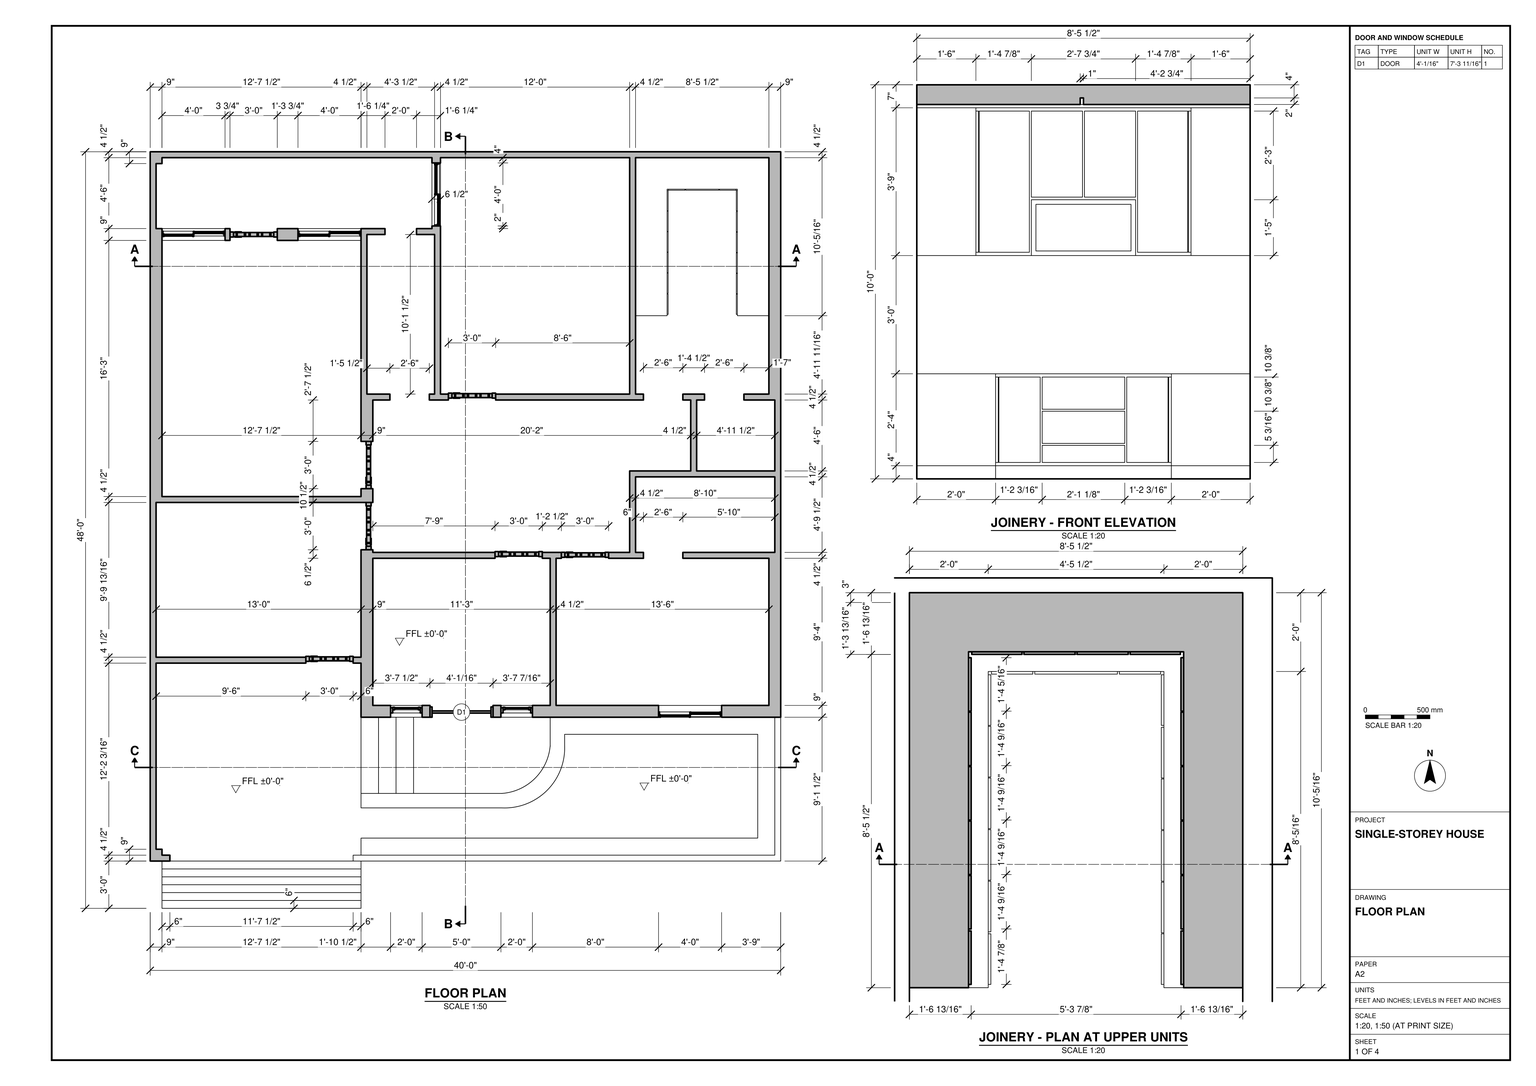
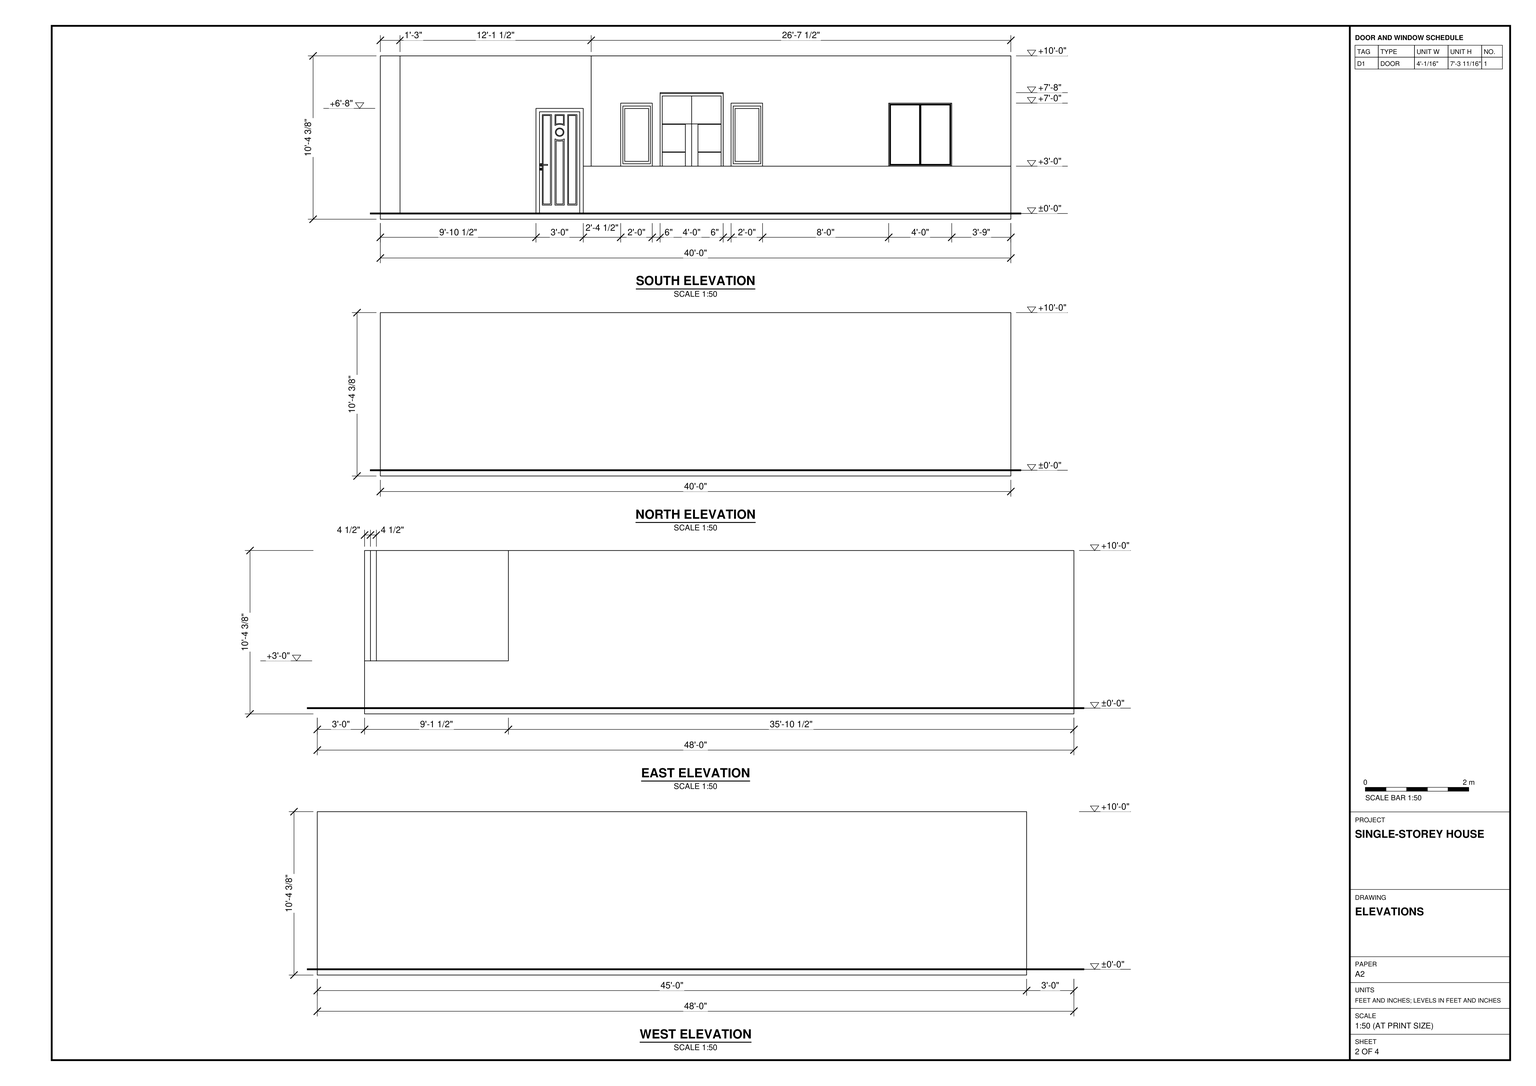
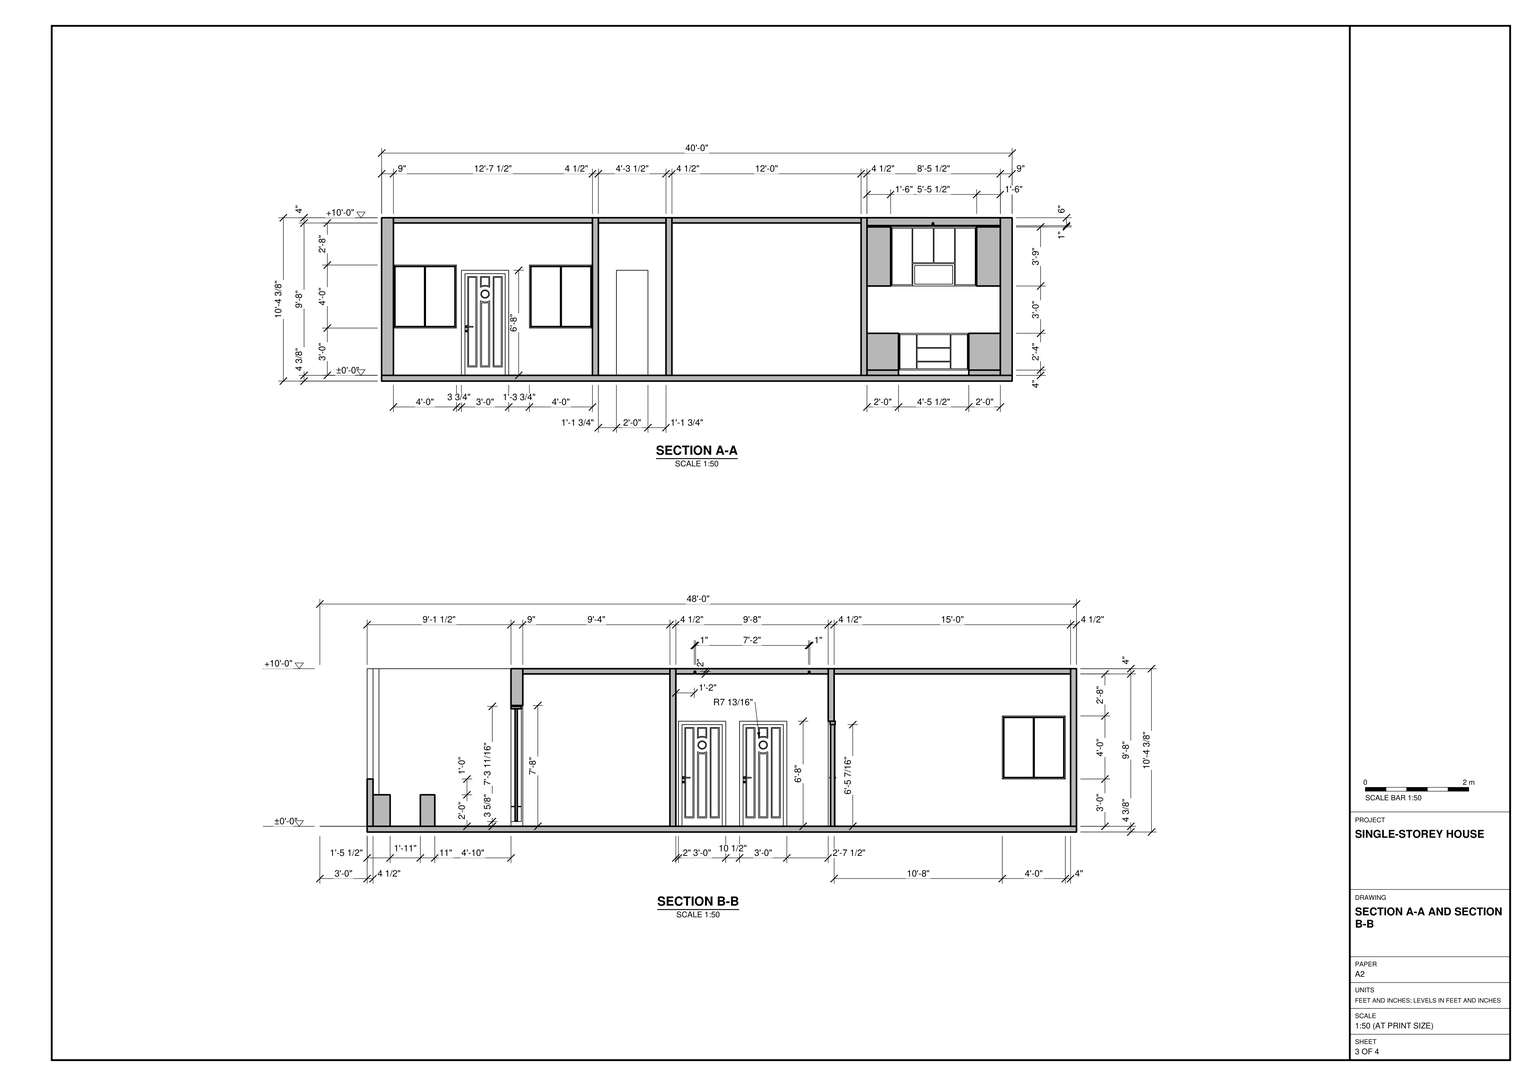
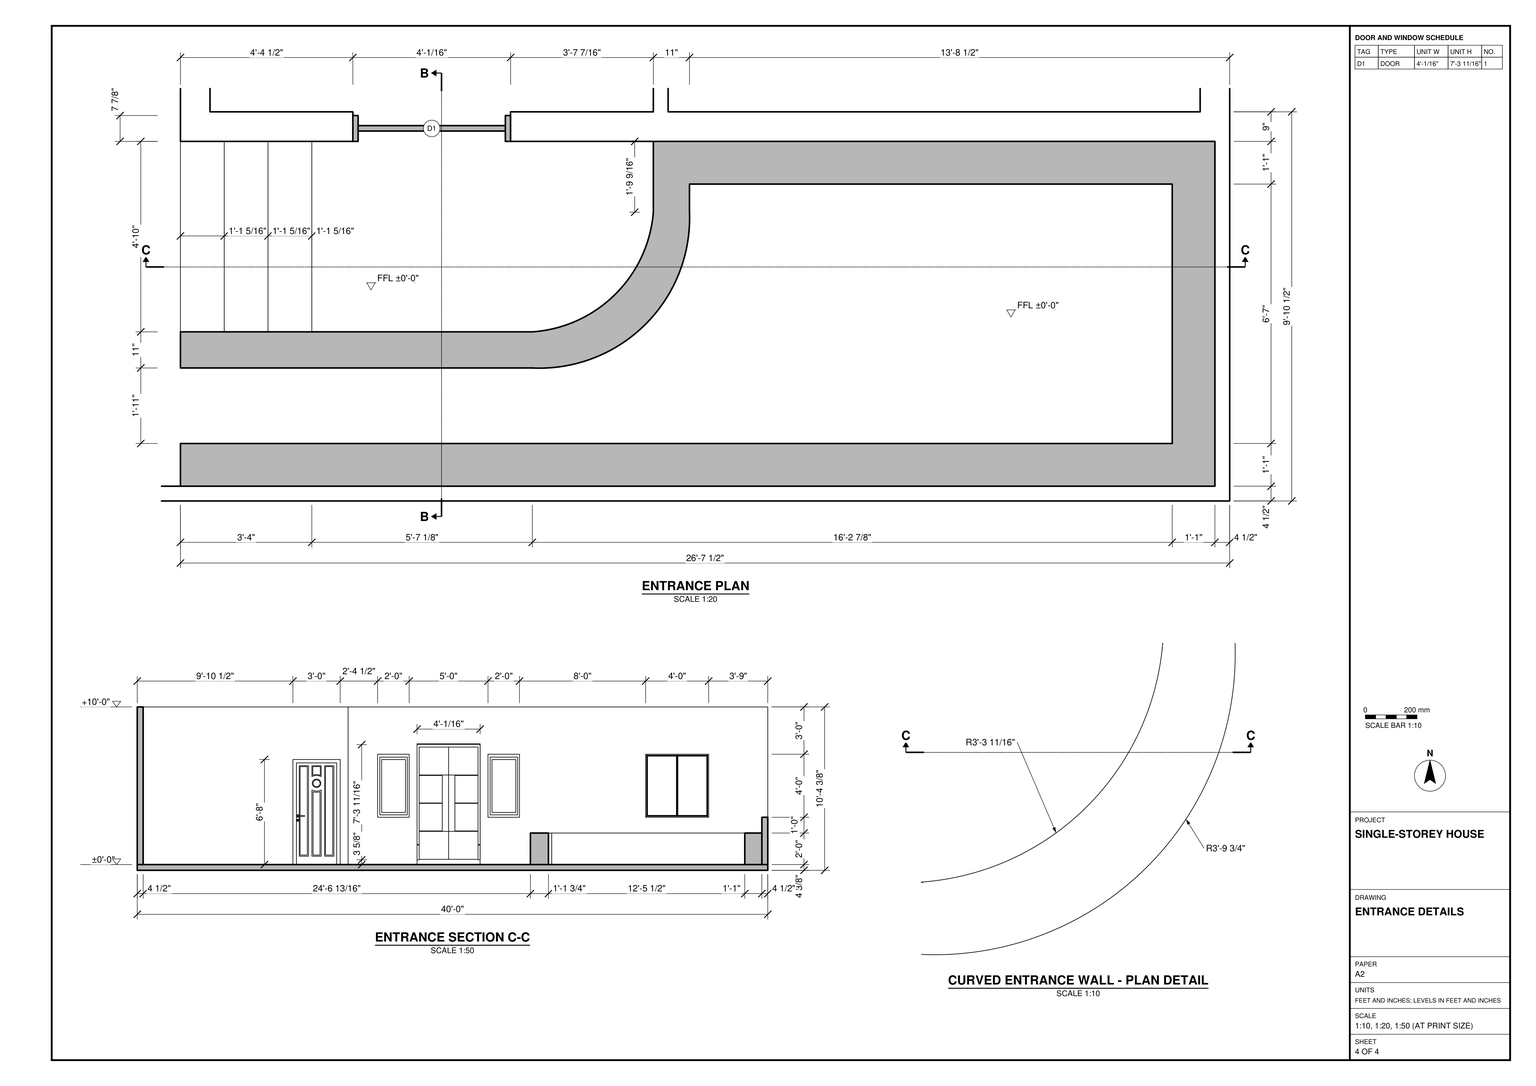
Build the house in SketchUp from task_files/diagram_01.pdf. Work in feet and inches. The overall dimensions, including the entry steps, are 40'-0" east to west, 48'-0" north to south and 10'-4 3/8" from the underside of the floor slab to the top of the roof. Use ±0'-0" as the finished floor level for the single storey.

Lay out the exterior walls and interior partitions from the floor plan, following the marked wall thicknesses rather than using one thickness throughout. Preserve the central circulation space, the rooms opening off it and the smaller compartments along the east side. Model the floor slab and flat roof slab using the sections. At the south entrance, include the steps on the west side and the low enclosure with its curved return. Fit the doors and framed window units to their openings, using the plan for placement and the elevations and sections for sill and head heights.

Build the joinery in the northeast room. Use the upper-unit plan for its U-shaped footprint and the front elevation for the upper cupboards, clear space above the base units and central drawer stack. Keep walls, slabs, roof and each furniture or joinery piece in separate groups or components, and use components for repeated parts. Decor and loose items shown may be represented by any suitable library components. Save one SketchUp model as output_files/single_storey_house_with_u_shaped_joinery.skp.

# SketchUp Ruby script. Lengths in inches.
U = 1.inch
M = Sketchup.active_model
def pt(a) = Geom::Point3d.new(a.map { |v| v * U })
def face(e, loops, mat)
  f = e.add_face(loops[0].map { |a| pt(a) })
  loops[1..].each { |l| e.add_face(l.map { |a| pt(a) }).erase! }
  f.material = f.back_material = mat if mat
  f
end
# faces: each face lists its corners as indices into pts; further lists are holes
def faces(e, pts, list, mat = nil) = list.each { |f| face(e, (f[0].is_a?(Array) ? f : [f]).map { |l| l.map { |i| pts[i] } }, mat) }
# xy, xz, yz: faces in a plane at the given z, y or x. An outline is a flat list of corners, or four numbers for a rectangle; further outlines are holes
def ring(l) = l.size == 4 ? [[l[0], l[1]], [l[2], l[1]], [l[2], l[3]], [l[0], l[3]]] : l.each_slice(2).to_a
def flat(e, list, mat, &to3) = list.each { |f| face(e, (f[0].is_a?(Array) ? f : [f]).map { |l| ring(l).map { |u, v| to3.(u, v) } }, mat) }
def xy(e, z, list, mat = nil) = flat(e, list, mat) { |x, y| [x, y, z] }
def xz(e, y, list, mat = nil) = flat(e, list, mat) { |x, z| [x, y, z] }
def yz(e, x, list, mat = nil) = flat(e, list, mat) { |y, z| [x, y, z] }
def lines(e, pts, list) = list.each { |a, b| e.add_line(pt(pts[a]), pt(pts[b])) }
# prism: a flat outline (further loops are holes) pulled along v
def prism(e, loops, v, mat = nil)
  f = face(e, loops, mat); d = Geom::Vector3d.new(v.map { |x| x * U })
  f.pushpull(f.normal.samedirection?(d) ? d.length : -d.length)
end
def box(e, o, s, mat = nil) = prism(e, [[o, [o[0] + s[0], o[1], o[2]], [o[0] + s[0], o[1] + s[1], o[2]], [o[0], o[1] + s[1], o[2]]]], [0, 0, s[2]], mat)
def at(x, y, z, deg = 0) = Geom::Transformation.translation(pt([x, y, z])) * Geom::Transformation.rotation(ORIGIN, Z_AXIS, deg.degrees)
def axes(o, x, y, z) = Geom::Transformation.new([*x, 0, *y, 0, *z, 0, *pt(o).to_a, 1])
def part(name) = M.definitions.add(name)
# library, detail: a bought-in or finely detailed component or shape, given as its bounding box
def library(name, o, s) = part(name).tap { |d| box(d.entities, o, s) }
def detail(e, o, s) = box(e.add_group.entities, o, s)
def put(e, d, t, mat = nil) = e.add_instance(d, t).tap { |i| i.material = mat if mat }
def group(e, t, mat = nil) = e.add_group.tap { |g| g.transformation = t; g.material = mat if mat }.entities
root = M.entities
M.materials.add("[0128_White]1").color = [255, 255, 255]
c1 = library("Double Door-006",[0,-7.875,0],[59.06,7.875,92.52])
c2 = library("door58",[0,0,0],[34.0625,4.69,80])
c3 = library("PENTEK_RP+Fineline+50S_Sliding_Door+(1)",[0,-2.27,-0.09],[99.27,4.05,99.27])
c4 = library("Group\#35",[29.18,0,0],[33.81,4.33,51.18])
c5 = library("Group\#7",[-0.5,-0.5,-0.1],[168.5,89,0.2])
c6 = library("Group\#8",[-0.5,-0.5,-0.1],[33.5,27,0.2])
c7 = library("Group\#5",[0,0,0],[101.5,120.3,28])
c8 = library("Group\#3",[0,0,0],[101.5,120.3,45])
c9 = library("Group\#11",[-0.5,-0.5,-6],[102.5,181,6])
xy(root,0,[[9,0,160.5,6],[9,6,160.5,12],[9,12,160.5,18],[9,18,160.5,24],[9,24,160.5,30],
  [9,30,160.5,36],[160.5,40.5,475.5,40.5,475.5,145.5,304.5,145.5,304.5,123.9375,315.5,123.9375,315.5,132.5,462.5,132.5,462.5,53.5,160.5,53.5],[273.77,86.84,273.15,86.85,272.53,86.87,271.92,86.91,271.3,86.95,270.68,87.01,270.07,87.09,269.45,87.17,268.84,87.27,268.23,87.38,267.625,87.5,268.19,87.54,268.76,87.59,269.33,87.65,269.9,87.72,270.46,87.8,271.03,87.88,271.59,87.97,272.15,88.07,272.71,88.18,273.83,88.42,274.38,88.55,274.93,88.69,275.49,88.84,276.03,89,276.58,89.16,277.125,89.33,277.67,89.51,278.21,89.7,278.74,89.89,279.28,90.1,279.81,90.31,280.33,90.52,280.86,90.75,281.38,90.98,281.9,91.22,282.92,91.72,283.43,91.99,284.43,92.53,285.41,93.11,285.9,93.41,286.38,93.71,286.86,94.02,287.33,94.34,288.27,95,288.72,95.34,289.18,95.68,289.63,96.03,290.07,96.39,290.51,96.76,290.94,97.13,291.8,97.89,292.21,98.28,292.625,98.67,293.03,99.07,293.43,99.48,293.82,99.89,294.21,100.3125,294.59,100.73,294.97,101.16,295.34,101.6,295.7,102.04,296.0625,102.48,296.41,102.93,296.76,103.39,297.09,103.85,297.42,104.3125,297.75,104.78,298.07,105.26,298.375,105.73,298.68,106.22,298.98,106.7,299.27,107.2,299.55,107.69,299.83,108.19,300.09,108.69,300.61,109.71,300.86,110.23,301.09,110.75,301.33,111.27,301.55,111.79,301.77,112.32,301.97,112.85,302.18,113.38,302.56,114.46,302.73,115,302.9,115.55,303.07,116.09,303.37,117.19,303.51,117.75,303.64,118.3,303.76,118.86,303.875,119.42,303.98,119.98,304.08,120.54,304.17,121.1,304.25,121.67,304.33,122.23,304.45,123.37,304.5,123.9375,304.61,123.33,304.72,122.72,304.81,122.11,304.88,121.49,304.95,120.875,305,120.26,305.04,119.64,305.07,119.02,305.09,118.4,305.09,117.78,305.08,117.16,305.0625,116.54,305.03,115.93,304.98,115.31,304.92,114.69,304.85,114.08,304.77,113.46,304.68,112.85,304.57,112.24,304.45,111.63,304.32,111.03,304.18,110.42,304.02,109.82,303.68,108.64,303.28,107.46,303.07,106.88,302.84,106.3,302.61,105.73,302.36,105.16,302.1,104.6,301.83,104.04,301.55,103.49,300.95,102.41,300.63,101.87,300.31,101.35,299.97,100.82,299.63,100.3125,299.27,99.8,298.91,99.3,298.53,98.8125,298.15,98.33,297.75,97.85,297.35,97.38,296.93,96.92,296.51,96.47,296.08,96.02,295.64,95.59,295.1875,95.16,294.73,94.74,294.26,94.34,293.79,93.9375,293.31,93.55,292.82,93.17,292.32,92.8,291.82,92.4375,291.31,92.09,290.79,91.75,290.27,91.42,289.73,91.1,289.2,90.79,288.1,90.21,287.55,89.94,286.99,89.67,286.42,89.42,285.85,89.18,285.28,88.95,284.7,88.73,284.12,88.52,283.53,88.33,282.9375,88.14,282.34,87.97,281.74,87.81,281.14,87.66,280.54,87.53,279.93,87.4,279.32,87.29,278.71,87.19,278.1,87.1,277.48,87.03,276.87,86.97,276.25,86.91,275.63,86.875,275.01,86.85,274.39,86.84],[160.5,87.5,173.83,145.5],[173.83,87.5,187.17,145.5],
  [187.17,87.5,200.5,145.5]])
xy(root,24,[[160.5,40.5,475.5,40.5,475.5,145.5,304.5,145.5,304.5,123.9375,304.45,123.37,304.33,122.23,304.25,121.67,304.17,121.1,304.08,120.54,303.98,119.98,303.875,119.42,303.76,118.86,303.64,118.3,303.51,117.75,303.37,117.19,303.07,116.09,302.9,115.55,302.73,115,302.56,114.46,302.18,113.38,301.97,112.85,301.77,112.32,301.55,111.79,301.33,111.27,301.09,110.75,300.86,110.23,300.61,109.71,300.09,108.69,299.83,108.19,299.55,107.69,299.27,107.2,298.98,106.7,298.68,106.22,298.375,105.73,298.07,105.26,297.75,104.78,297.42,104.3125,297.09,103.85,296.76,103.39,296.41,102.93,296.0625,102.48,295.7,102.04,295.34,101.6,294.97,101.16,294.59,100.73,294.21,100.3125,293.82,99.89,293.43,99.48,293.03,99.07,292.625,98.67,292.21,98.28,291.8,97.89,290.94,97.13,290.51,96.76,290.07,96.39,289.63,96.03,289.18,95.68,288.72,95.34,288.27,95,287.33,94.34,286.86,94.02,286.38,93.71,285.9,93.41,285.41,93.11,284.43,92.53,283.43,91.99,282.92,91.72,281.9,91.22,281.38,90.98,280.86,90.75,280.33,90.52,279.81,90.31,279.28,90.1,278.74,89.89,278.21,89.7,277.67,89.51,277.125,89.33,276.58,89.16,276.03,89,275.49,88.84,274.93,88.69,274.38,88.55,273.83,88.42,272.71,88.18,272.15,88.07,271.59,87.97,271.03,87.88,270.46,87.8,269.9,87.72,269.33,87.65,268.76,87.59,268.19,87.54,267.625,87.5,160.5,87.5,160.5,76.5,267.625,76.5,268.39,76.47,269.15,76.45,269.92,76.45,270.69,76.46,271.45,76.48,272.22,76.51,272.98,76.56,273.74,76.62,274.5,76.69,275.26,76.78,276.02,76.875,276.78,76.99,277.54,77.11,278.29,77.24,279.04,77.39,279.79,77.55,280.53,77.73,281.28,77.91,282.02,78.11,282.75,78.32,283.48,78.54,284.21,78.78,284.9375,79.03,285.66,79.29,286.37,79.56,287.08,79.84,287.79,80.14,288.49,80.44,289.19,80.76,289.875,81.09,290.56,81.43,291.24,81.79,291.91,82.15,292.58,82.53,293.24,82.91,293.89,83.3125,294.54,83.72,295.18,84.14,295.8125,84.57,296.44,85.01,297.06,85.46,297.67,85.92,298.27,86.39,298.87,86.875,299.45,87.37,300.03,87.87,300.6,88.38,301.16,88.9,301.72,89.43,302.26,89.97,302.79,90.51,303.32,91.07,304.34,92.21,304.84,92.79,305.32,93.38,305.8,93.98,306.27,94.59,306.73,95.2,307.17,95.82,307.61,96.45,308.45,97.73,308.85,98.38,309.24,99.04,309.625,99.7,310,100.37,310.36,101.05,310.7,101.73,311.04,102.42,311.37,103.11,311.68,103.81,311.98,104.51,312.27,105.22,312.55,105.93,312.8125,106.65,313.07,107.37,313.31,108.1,313.54,108.83,313.76,109.5625,313.96,110.3,314.15,111.04,314.33,111.78,314.5,112.53,314.66,113.28,314.8,114.03,314.93,114.79,315.05,115.54,315.15,116.3,315.25,117.0625,315.32,117.82,315.39,118.58,315.45,119.35,315.49,120.11,315.53,121.64,315.53,122.41,315.52,123.17,315.5,123.9375,315.5,132.5,462.5,132.5,462.5,53.5,160.5,53.5]])
xy(root,120,[[4.5,517.5,214.5,571.5]])
xz(root,40.5,[[160.5,0,475.5,24]])
xz(root,53.5,[[160.5,0,462.5,24]])
xz(root,76.45,[[269.15,0,269.92,24]])
xz(root,76.5,[[160.5,0,267.625,24]])
xz(root,87.5,[[160.5,0,267.625,24]])
xz(root,132.5,[[315.5,0,462.5,24]])
xz(root,145.5,[[304.5,0,475.5,24]])
yz(root,160.5,[[40.5,0,53.5,24],[76.5,0,87.5,24]])
yz(root,304.5,[[123.9375,0,145.5,24]])
yz(root,315.5,[[123.9375,0,132.5,24]])
yz(root,315.53,[[121.64,0,122.41,24]])
yz(root,462.5,[[53.5,0,132.5,24]])
yz(root,475.5,[[40.5,0,145.5,24]])
# 98 loose lines left out
p = [[269.92,76.45,0],[270.69,76.46,0],[270.69,76.46,24],[269.92,76.45,24],[267.625,76.5,0],[268.39,76.47,0],
  [268.39,76.47,24],[267.625,76.5,24],[269.15,76.45,0],[269.15,76.45,24],[271.45,76.48,0],[271.45,76.48,24],
  [272.22,76.51,0],[272.22,76.51,24],[272.98,76.56,0],[272.98,76.56,24],[273.74,76.62,0],[273.74,76.62,24],
  [274.5,76.69,0],[274.5,76.69,24],[275.26,76.78,0],[275.26,76.78,24],[276.02,76.875,0],[276.02,76.875,24],
  [276.78,76.99,0],[276.78,76.99,24],[277.54,77.11,0],[277.54,77.11,24],[278.29,77.24,0],[278.29,77.24,24],
  [279.04,77.39,0],[279.04,77.39,24],[279.79,77.55,0],[279.79,77.55,24],[280.53,77.73,0],[280.53,77.73,24],
  [281.28,77.91,0],[281.28,77.91,24],[282.02,78.11,0],[282.02,78.11,24],[282.75,78.32,0],[282.75,78.32,24],
  [283.48,78.54,0],[283.48,78.54,24],[284.21,78.78,0],[284.21,78.78,24],[284.9375,79.03,0],[284.9375,79.03,24],
  [285.66,79.29,0],[285.66,79.29,24],[286.37,79.56,0],[286.37,79.56,24],[287.08,79.84,0],[287.08,79.84,24],
  [287.79,80.14,0],[287.79,80.14,24],[288.49,80.44,0],[288.49,80.44,24],[289.19,80.76,0],[289.19,80.76,24],
  [289.875,81.09,0],[289.875,81.09,24],[290.56,81.43,0],[290.56,81.43,24],[291.24,81.79,0],[291.24,81.79,24],
  [291.91,82.15,0],[291.91,82.15,24],[292.58,82.53,0],[292.58,82.53,24],[293.24,82.91,0],[293.24,82.91,24],
  [293.89,83.3125,0],[293.89,83.3125,24],[294.54,83.72,0],[294.54,83.72,24],[295.18,84.14,0],[295.18,84.14,24],
  [295.8125,84.57,0],[295.8125,84.57,24],[296.44,85.01,0],[296.44,85.01,24],[297.06,85.46,0],[297.06,85.46,24],
  [297.67,85.92,0],[297.67,85.92,24],[298.27,86.39,0],[298.27,86.39,24],[298.87,86.875,0],[298.87,86.875,24],
  [299.45,87.37,0],[299.45,87.37,24],[300.03,87.87,0],[300.03,87.87,24],[268.19,87.54,0],[267.625,87.5,0],
  [267.625,87.5,24],[268.19,87.54,24],[268.76,87.59,0],[268.76,87.59,24],[269.33,87.65,0],[269.33,87.65,24],
  [269.9,87.72,0],[269.9,87.72,24],[270.46,87.8,0],[270.46,87.8,24],[271.03,87.88,0],[271.03,87.88,24],
  [271.59,87.97,0],[271.59,87.97,24],[300.6,88.38,0],[300.6,88.38,24],[272.15,88.07,0],[272.15,88.07,24],
  [272.71,88.18,0],[272.71,88.18,24],[273.27,88.3,0],[273.27,88.3,24],[273.83,88.42,0],[273.83,88.42,24],
  [274.38,88.55,0],[274.38,88.55,24],[301.16,88.9,0],[301.16,88.9,24],[274.93,88.69,0],[274.93,88.69,24],
  [275.49,88.84,0],[275.49,88.84,24],[276.03,89,0],[276.03,89,24],[301.72,89.43,0],[301.72,89.43,24],
  [276.58,89.16,0],[276.58,89.16,24],[277.125,89.33,0],[277.125,89.33,24],[277.67,89.51,0],[277.67,89.51,24],
  [302.26,89.97,0],[302.26,89.97,24],[278.21,89.7,0],[278.21,89.7,24],[278.74,89.89,0],[278.74,89.89,24],
  [279.28,90.1,0],[279.28,90.1,24],[302.79,90.51,0],[302.79,90.51,24],[279.81,90.31,0],[279.81,90.31,24],
  [280.33,90.52,0],[280.33,90.52,24],[280.86,90.75,0],[280.86,90.75,24],[303.32,91.07,0],[303.32,91.07,24],
  [281.38,90.98,0],[281.38,90.98,24],[281.9,91.22,0],[281.9,91.22,24],[303.83,91.64,0],[303.83,91.64,24],
  [282.41,91.47,0],[282.41,91.47,24],[282.92,91.72,0],[282.92,91.72,24],[304.34,92.21,0],[304.34,92.21,24],
  [283.43,91.99,0],[283.43,91.99,24],[283.93,92.26,0],[283.93,92.26,24],[304.84,92.79,0],[304.84,92.79,24],
  [284.43,92.53,0],[284.43,92.53,24],[284.92,92.82,0],[284.92,92.82,24],[285.41,93.11,0],[285.41,93.11,24],
  [305.32,93.38,0],[305.32,93.38,24],[285.9,93.41,0],[285.9,93.41,24],[286.38,93.71,0],[286.38,93.71,24],
  [305.8,93.98,0],[305.8,93.98,24],[286.86,94.02,0],[286.86,94.02,24],[287.33,94.34,0],[287.33,94.34,24],
  [306.27,94.59,0],[306.27,94.59,24],[287.8,94.67,0],[287.8,94.67,24],[306.73,95.2,0],[306.73,95.2,24],
  [288.27,95,0],[288.27,95,24],[288.72,95.34,0],[288.72,95.34,24],[307.17,95.82,0],[307.17,95.82,24],
  [289.18,95.68,0],[289.18,95.68,24],[289.63,96.03,0],[289.63,96.03,24],[307.61,96.45,0],[307.61,96.45,24],
  [290.07,96.39,0],[290.07,96.39,24],[290.51,96.76,0],[290.51,96.76,24],[308.03,97.09,0],[308.03,97.09,24],
  [290.94,97.13,0],[290.94,97.13,24],[291.37,97.51,0],[291.37,97.51,24],[308.45,97.73,0],[308.45,97.73,24],
  [291.8,97.89,0],[291.8,97.89,24],[308.85,98.38,0],[308.85,98.38,24],[292.21,98.28,0],[292.21,98.28,24],
  [292.625,98.67,0],[292.625,98.67,24],[309.24,99.04,0],[309.24,99.04,24],[293.03,99.07,0],[293.03,99.07,24],
  [309.625,99.7,0],[309.625,99.7,24],[293.43,99.48,0],[293.43,99.48,24],[293.82,99.89,0],[293.82,99.89,24],
  [310,100.37,0],[310,100.37,24],[294.21,100.3125,0],[294.21,100.3125,24],[294.59,100.73,0],[294.59,100.73,24],
  [310.36,101.05,0],[310.36,101.05,24],[294.97,101.16,0],[294.97,101.16,24],[310.7,101.73,0],[310.7,101.73,24],
  [295.34,101.6,0],[295.34,101.6,24],[295.7,102.04,0],[295.7,102.04,24],[311.04,102.42,0],[311.04,102.42,24],
  [296.0625,102.48,0],[296.0625,102.48,24],[311.37,103.11,0],[311.37,103.11,24],[296.41,102.93,0],[296.41,102.93,24],
  [296.76,103.39,0],[296.76,103.39,24],[311.68,103.81,0],[311.68,103.81,24],[297.09,103.85,0],[297.09,103.85,24],
  [297.42,104.3125,0],[297.42,104.3125,24],[311.98,104.51,0],[311.98,104.51,24],[297.75,104.78,0],[297.75,104.78,24],
  [312.27,105.22,0],[312.27,105.22,24],[298.07,105.26,0],[298.07,105.26,24],[312.55,105.93,0],[312.55,105.93,24],
  [298.375,105.73,0],[298.375,105.73,24],[298.68,106.22,0],[298.68,106.22,24],[312.8125,106.65,0],[312.8125,106.65,24],
  [298.98,106.7,0],[298.98,106.7,24],[299.27,107.2,0],[299.27,107.2,24],[313.07,107.37,0],[313.07,107.37,24],
  [299.55,107.69,0],[299.55,107.69,24],[313.31,108.1,0],[313.31,108.1,24],[299.83,108.19,0],[299.83,108.19,24],
  [313.54,108.83,0],[313.54,108.83,24],[300.09,108.69,0],[300.09,108.69,24],[300.35,109.2,0],[300.35,109.2,24],
  [313.76,109.5625,0],[313.76,109.5625,24],[300.61,109.71,0],[300.61,109.71,24],[313.96,110.3,0],[313.96,110.3,24],
  [300.86,110.23,0],[300.86,110.23,24],[301.09,110.75,0],[301.09,110.75,24],[314.15,111.04,0],[314.15,111.04,24],
  [301.33,111.27,0],[301.33,111.27,24],[314.33,111.78,0],[314.33,111.78,24],[301.55,111.79,0],[301.55,111.79,24],
  [301.77,112.32,0],[301.77,112.32,24],[314.5,112.53,0],[314.5,112.53,24],[301.97,112.85,0],[301.97,112.85,24],
  [314.66,113.28,0],[314.66,113.28,24],[302.18,113.38,0],[302.18,113.38,24],[314.8,114.03,0],[314.8,114.03,24],
  [302.37,113.92,0],[302.37,113.92,24],[302.56,114.46,0],[302.56,114.46,24],[314.93,114.79,0],[314.93,114.79,24],
  [302.73,115,0],[302.73,115,24],[315.05,115.54,0],[315.05,115.54,24],[302.9,115.55,0],[302.9,115.55,24],
  [303.07,116.09,0],[303.07,116.09,24],[315.15,116.3,0],[315.15,116.3,24],[303.22,116.64,0],[303.22,116.64,24],
  [315.25,117.0625,0],[315.25,117.0625,24],[303.37,117.19,0],[303.37,117.19,24],[315.32,117.82,0],[315.32,117.82,24],
  [303.51,117.75,0],[303.51,117.75,24],[303.64,118.3,0],[303.64,118.3,24],[315.39,118.58,0],[315.39,118.58,24],
  [303.76,118.86,0],[303.76,118.86,24],[315.45,119.35,0],[315.45,119.35,24],[303.875,119.42,0],[303.875,119.42,24],
  [315.49,120.11,0],[315.49,120.11,24],[303.98,119.98,0],[303.98,119.98,24],[304.08,120.54,0],[304.08,120.54,24],
  [315.51,120.875,0],[315.51,120.875,24],[304.17,121.1,0],[304.17,121.1,24],[315.53,121.64,0],[315.53,121.64,24],
  [304.25,121.67,0],[304.25,121.67,24],[304.33,122.23,0],[304.33,122.23,24],[304.39,122.8,0],[304.39,122.8,24],
  [315.53,122.41,0],[315.52,123.17,0],[315.52,123.17,24],[315.53,122.41,24],[304.45,123.37,0],[304.45,123.37,24],
  [315.5,123.9375,0],[315.5,123.9375,24],[304.5,123.9375,0],[304.5,123.9375,24]]
faces(root,p,[[0,1,2,3],[4,5,6,7],[5,8,9,6],[1,10,11,2],[10,12,13,11],[12,14,15,13],[14,16,17,15],[16,18,19,17],
  [18,20,21,19],[20,22,23,21],[22,24,25,23],[24,26,27,25],[26,28,29,27],[28,30,31,29],[30,32,33,31],[32,34,35,33],
  [34,36,37,35],[36,38,39,37],[38,40,41,39],[40,42,43,41],[42,44,45,43],[44,46,47,45],[46,48,49,47],[48,50,51,49],
  [50,52,53,51],[52,54,55,53],[54,56,57,55],[56,58,59,57],[58,60,61,59],[60,62,63,61],[62,64,65,63],[64,66,67,65],
  [66,68,69,67],[68,70,71,69],[70,72,73,71],[72,74,75,73],[74,76,77,75],[76,78,79,77],[78,80,81,79],[80,82,83,81],
  [82,84,85,83],[84,86,87,85],[86,88,89,87],[88,90,91,89],[90,92,93,91],[94,95,96,97],[98,94,97,99],[100,98,99,101],
  [102,100,101,103],[104,102,103,105],[106,104,105,107],[108,106,107,109],[92,110,111,93],[112,108,109,113],[114,112,113,115],[116,114,115,117],
  [118,116,117,119],[120,118,119,121],[110,122,123,111],[124,120,121,125],[126,124,125,127],[128,126,127,129],[122,130,131,123],[132,128,129,133],
  [134,132,133,135],[136,134,135,137],[130,138,139,131],[140,136,137,141],[142,140,141,143],[144,142,143,145],[138,146,147,139],[148,144,145,149],
  [150,148,149,151],[152,150,151,153],[146,154,155,147],[156,152,153,157],[158,156,157,159],[154,160,161,155],[162,158,159,163],[164,162,163,165],
  [160,166,167,161],[168,164,165,169],[170,168,169,171],[166,172,173,167],[174,170,171,175],[176,174,175,177],[178,176,177,179],[172,180,181,173],
  [182,178,179,183],[184,182,183,185],[180,186,187,181],[188,184,185,189],[190,188,189,191],[186,192,193,187],[194,190,191,195],[192,196,197,193],
  [198,194,195,199],[200,198,199,201],[196,202,203,197],[204,200,201,205],[206,204,205,207],[202,208,209,203],[210,206,207,211],[212,210,211,213],
  [208,214,215,209],[216,212,213,217],[218,216,217,219],[214,220,221,215],[222,218,219,223],[220,224,225,221],[226,222,223,227],[228,226,227,229],
  [224,230,231,225],[232,228,229,233],[230,234,235,231],[236,232,233,237],[238,236,237,239],[234,240,241,235],[242,238,239,243],[244,242,243,245],
  [240,246,247,241],[248,244,245,249],[246,250,251,247],[252,248,249,253],[254,252,253,255],[250,256,257,251],[258,254,255,259],[256,260,261,257],
  [262,258,259,263],[264,262,263,265],[260,266,267,261],[268,264,265,269],[270,268,269,271],[266,272,273,267],[274,270,271,275],[272,276,277,273],
  [278,274,275,279],[276,280,281,277],[282,278,279,283],[284,282,283,285],[280,286,287,281],[288,284,285,289],[290,288,289,291],[286,292,293,287],
  [294,290,291,295],[292,296,297,293],[298,294,295,299],[296,300,301,297],[302,298,299,303],[304,302,303,305],[300,306,307,301],[308,304,305,309],
  [306,310,311,307],[312,308,309,313],[314,312,313,315],[310,316,317,311],[318,314,315,319],[316,320,321,317],[322,318,319,323],[324,322,323,325],
  [320,326,327,321],[328,324,325,329],[326,330,331,327],[332,328,329,333],[330,334,335,331],[336,332,333,337],[338,336,337,339],[334,340,341,335],
  [342,338,339,343],[340,344,345,341],[346,342,343,347],[348,346,347,349],[344,350,351,345],[352,348,349,353],[350,354,355,351],[356,352,353,357],
  [354,358,359,355],[360,356,357,361],[362,360,361,363],[358,364,365,359],[366,362,363,367],[364,368,369,365],[370,366,367,371],[368,372,373,369],
  [374,370,371,375],[376,374,375,377],[372,378,379,373],[380,376,377,381],[378,382,383,379],[384,380,381,385],[386,384,385,387],[388,386,387,389],
  [390,391,392,393],[394,388,389,395],[391,396,397,392],[398,394,395,399]])
put(root,c1,axes([213,153.375,3.625],[0.81337,0,0],[0,1,0],[0,0,0.94789]))
put(root,c2,axes([60.75,510.68,0],[1.05686,0,0],[0,1,0],[0,0,1]))
put(root,c2,axes([227,388.02,0],[1.05686,0,0],[0,1,0],[0,0,1]))
put(root,c2,axes([262.5,267.38,0],[1.05686,0,0],[0,1,0],[0,0,1]))
put(root,c2,axes([313,266.84,0],[1.05686,0,0],[0,1,0],[0,0,1]))
put(root,c2,axes([168.6,319.5,0],[0,1.05686,0],[-1,0,0],[0,0,1]))
put(root,c2,axes([168.6,273,0],[0,1.05686,0],[-1,0,0],[0,0,1]))
put(root,c2,axes([118.5,187.625,0],[1.05686,0,0],[0,1,0],[0,0,1]))
put(root,c3,axes([387,147.77,36.04],[0.48352,0,0],[0,1,0],[0,0,0.48352]))
put(root,c3,axes([112.5,513.75,36.04],[0.48352,0,0],[0,1,0],[0,0,0.48352]))
put(root,c3,axes([9,513.75,36.04],[0.48352,0,0],[0,1,0],[0,0,0.48352]))
put(root,c3,axes([218.28,519.5,36.04],[0,0.48352,0],[-1,0,0],[0,0,0.48352]))
g1 = group(root,at(0,36,0))
xy(g1,0,[[0,0,0,540,480,540,480,0,154.5,0,154.5,4.5,475.5,4.5,475.5,109.5,261,109.5,261,118.5,304.5,118.5,304.5,230.5,298.5,230.5,298.5,235,313,235,313,230.5,309,230.5,309,118.5,471,118.5,471,230.5,405.5,230.5,405.5,235,475.5,235,475.5,292.5,369.5,292.5,369.5,235,375.5,235,375.5,230.5,349,230.5,349,235,365,235,365,297,411.5,297,411.5,351,405.5,351,405.5,355.5,422,355.5,422,351,416,351,416,297,475.5,297,475.5,351,452,351,452,355.5,471,355.5,471,535.5,369.5,535.5,369.5,355.5,375.5,355.5,375.5,351,263,351,263,355.5,365,355.5,365,535.5,221,535.5,221,355.5,227,355.5,227,351,212.5,351,212.5,355.5,216.5,355.5,216.5,477,202.75,477,202.75,481.5,214.5,481.5,214.5,535.5,9,535.5,9,531,4.5,531,4.5,481.5,60.75,481.5,60.75,472.5,9,472.5,9,277.5,160.5,277.5,160.5,283.5,169.5,283.5,169.5,273,4.5,273,4.5,155.19,118.5,155.19,118.5,150.69,4.5,150.69,4.5,9,9,9,9,4.5,15,4.5,15,0],[160.5,109.5,160.5,150.69,154.5,150.69,154.5,155.19,160.5,155.19,160.5,237,169.5,237,169.5,235,262.5,235,262.5,230.5,169.5,230.5,169.5,118.5,213,118.5,213,109.5],[160.5,319.5,160.5,472.5,96.75,472.5,96.75,481.5,178.75,481.5,178.75,477,165,477,165,355.5,182.5,355.5,182.5,351,169.5,351,169.5,319.5]])
xy(g1,36,[[154.5,0,480,0,480,109.5,475.5,109.5,475.5,4.5,154.5,4.5],[183,109.5,207,118.5],[267,109.5,291,118.5],[387,109.5,435,118.5],[9,472.5,57,481.5],
  [112.5,472.5,160.5,481.5],[214.5,483.5,221,531.5]])
xy(g1,80,[[118.5,150.69,154.5,155.19],[262.5,230.5,298.5,235],[313,230.5,349,235],[375.5,230.5,405.5,235],[160.5,237,169.5,273],
  [160.5,283.5,169.5,319.5],[182.5,351,212.5,355.5],[227,351,263,355.5],[422,351,452,355.5],[60.75,472.5,96.75,481.5],
  [178.75,477,202.75,481.5]])
xy(g1,84,[[183,109.5,207,118.5],[267,109.5,291,118.5],[387,109.5,435,118.5],[9,472.5,57,481.5],[112.5,472.5,160.5,481.5],
  [214.5,483.5,221,531.5]])
xy(g1,87.0625,[[390.33,351,390.67,355.5]])
xy(g1,92,[[213,109.5,261,118.5]])
xy(g1,120,[[[0,0,15,0,15,4.5,9,4.5,9,9,4.5,9,4.5,150.69,160.5,150.69,160.5,109.5,480,109.5,480,540,0,540],[9,277.5,160.5,472.5],[221,355.5,365,535.5],[169.5,235,169.5,351,411.5,351,411.5,297,365,297,365,235],[4.5,155.19,160.5,273],[369.5,355.5,471,535.5],[309,118.5,471,230.5],[169.5,118.5,304.5,230.5],[4.5,481.5,4.5,531,9,531,9,535.5,214.5,535.5,214.5,481.5],[165,355.5,216.5,477],[369.5,235,475.5,292.5],[416,297,475.5,351]]])
xz(g1,0,[[0,0,15,120],[154.5,0,480,36]])
xz(g1,4.5,[[9,0,15,120],[154.5,0,475.5,36]])
xz(g1,9,[[4.5,0,9,120]])
xz(g1,109.5,[[[160.5,0,213,0,213,92,261,92,261,0,475.5,0,475.5,36,480,36,480,120,160.5,120],[387,36,435,84],[267,36,291,84],[183,36,207,84]]])
xz(g1,118.5,[[[169.5,0,169.5,120,304.5,120,304.5,0,261,0,261,92,213,92,213,0],[267,36,291,84],[183,36,207,84]],[[309,0,471,120],[387,36,435,84]]])
xz(g1,150.69,[[4.5,0,118.5,0,118.5,80,154.5,80,154.5,0,160.5,0,160.5,120,4.5,120]])
xz(g1,155.19,[[4.5,0,4.5,120,160.5,120,160.5,0,154.5,0,154.5,80,118.5,80,118.5,0]])
xz(g1,230.5,[[169.5,0,262.5,0,262.5,80,298.5,80,298.5,0,304.5,0,304.5,120,169.5,120],[309,0,313,0,313,80,349,80,349,0,375.5,0,375.5,80,405.5,80,405.5,0,471,0,471,120,309,120]])
xz(g1,235,[[169.5,0,169.5,120,365,120,365,0,349,0,349,80,313,80,313,0,298.5,0,298.5,80,262.5,80,262.5,0],[369.5,0,369.5,120,475.5,120,475.5,0,405.5,0,405.5,80,375.5,80,375.5,0]])
xz(g1,237,[[160.5,0,169.5,80]])
xz(g1,273,[[4.5,0,169.5,0,169.5,80,160.5,80,160.5,120,4.5,120]])
xz(g1,277.5,[[9,0,160.5,120]])
xz(g1,283.5,[[160.5,0,169.5,80]])
xz(g1,292.5,[[369.5,0,475.5,120]])
xz(g1,297,[[365,0,411.5,120],[416,0,475.5,120]])
xz(g1,319.5,[[160.5,0,169.5,80]])
xz(g1,351,[[169.5,0,182.5,0,182.5,80,212.5,80,212.5,0,227,0,227,80,263,80,263,0,375.5,0,375.5,80,375.72,80.26,375.95,80.53,376.18,80.78,376.66,81.28,376.91,81.53,377.16,81.77,377.41,82,377.93,82.46,378.2,82.68,378.47,82.89,378.74,83.11,379.02,83.3125,379.3,83.51,379.58,83.71,380.16,84.09,380.46,84.27,380.75,84.45,381.06,84.62,381.36,84.78,381.98,85.1,382.29,85.25,382.6,85.39,382.92,85.53,383.24,85.66,383.5625,85.78,383.89,85.9,384.21,86.02,384.54,86.13,385.2,86.33,385.54,86.42,386.21,86.58,386.55,86.66,386.89,86.72,387.23,86.79,387.91,86.89,388.26,86.93,388.6,86.97,388.94,87,389.64,87.04,389.98,87.06,390.33,87.0625,390.67,87.0625,391.02,87.06,391.36,87.04,392.06,87,392.4,86.97,392.74,86.93,393.09,86.89,393.77,86.79,394.11,86.72,394.45,86.66,394.79,86.58,395.46,86.42,395.8,86.33,396.46,86.13,396.79,86.02,397.11,85.9,397.4375,85.78,397.76,85.66,398.08,85.53,398.4,85.39,398.71,85.25,399.02,85.1,399.64,84.78,399.94,84.62,400.25,84.45,400.54,84.27,400.84,84.09,401.42,83.71,401.7,83.51,401.98,83.3125,402.26,83.11,402.53,82.89,402.8,82.68,403.07,82.46,403.59,82,403.84,81.77,404.09,81.53,404.34,81.28,404.82,80.78,405.05,80.53,405.28,80.26,405.5,80,405.5,0,411.5,0,411.5,120,169.5,120],[416,0,422,0,422,80,452,80,452,0,475.5,0,475.5,120,416,120]])
xz(g1,355.5,[[165,0,165,120,216.5,120,216.5,0,212.5,0,212.5,80,182.5,80,182.5,0],[221,0,221,120,365,120,365,0,263,0,263,80,227,80,227,0],[369.5,0,369.5,120,471,120,471,0,452,0,452,80,422,80,422,0,405.5,0,405.5,80,405.28,80.26,405.05,80.53,404.82,80.78,404.34,81.28,404.09,81.53,403.84,81.77,403.59,82,403.07,82.46,402.8,82.68,402.53,82.89,402.26,83.11,401.98,83.3125,401.7,83.51,401.42,83.71,400.84,84.09,400.54,84.27,400.25,84.45,399.94,84.62,399.64,84.78,399.02,85.1,398.71,85.25,398.4,85.39,398.08,85.53,397.76,85.66,397.4375,85.78,397.11,85.9,396.79,86.02,396.46,86.13,395.8,86.33,395.46,86.42,394.79,86.58,394.45,86.66,394.11,86.72,393.77,86.79,393.09,86.89,392.74,86.93,392.4,86.97,392.06,87,391.36,87.04,391.02,87.06,390.67,87.0625,390.33,87.0625,389.98,87.06,389.64,87.04,388.94,87,388.6,86.97,388.26,86.93,387.91,86.89,387.23,86.79,386.89,86.72,386.55,86.66,386.21,86.58,385.54,86.42,385.2,86.33,384.54,86.13,384.21,86.02,383.89,85.9,383.5625,85.78,383.24,85.66,382.92,85.53,382.6,85.39,382.29,85.25,381.98,85.1,381.36,84.78,381.06,84.62,380.75,84.45,380.46,84.27,380.16,84.09,379.58,83.71,379.3,83.51,379.02,83.3125,378.74,83.11,378.47,82.89,378.2,82.68,377.93,82.46,377.41,82,377.16,81.77,376.91,81.53,376.66,81.28,376.18,80.78,375.95,80.53,375.72,80.26,375.5,80,375.5,0]])
xz(g1,472.5,[[9,0,60.75,0,60.75,80,96.75,80,96.75,0,160.5,0,160.5,36,112.5,36,112.5,84,160.5,84,160.5,120,9,120,9,84,57,84,57,36,9,36]])
xz(g1,477,[[165,0,178.75,0,178.75,80,202.75,80,202.75,0,216.5,0,216.5,120,165,120]])
xz(g1,481.5,[[[4.5,0,4.5,120,214.5,120,214.5,0,202.75,0,202.75,80,178.75,80,178.75,0,96.75,0,96.75,80,60.75,80,60.75,0],[9,36,57,84],[112.5,36,160.5,84]]])
xz(g1,483.5,[[214.5,36,221,84]])
xz(g1,531,[[4.5,0,9,120]])
xz(g1,531.5,[[214.5,36,221,84]])
xz(g1,535.5,[[9,0,214.5,120],[221,0,365,120],[369.5,0,471,120]])
xz(g1,540,[[0,0,480,120]])
yz(g1,0,[[0,0,540,120]])
yz(g1,4.5,[[9,0,150.69,120],[155.19,0,273,120],[481.5,0,531,120]])
yz(g1,9,[[4.5,0,9,120],[277.5,0,472.5,0,472.5,36,481.5,36,481.5,84,472.5,84,472.5,120,277.5,120],[531,0,535.5,120]])
yz(g1,15,[[0,0,4.5,120]])
yz(g1,57,[[472.5,36,481.5,84]])
yz(g1,60.75,[[472.5,0,481.5,80]])
yz(g1,96.75,[[472.5,0,481.5,80]])
yz(g1,112.5,[[472.5,36,481.5,84]])
yz(g1,118.5,[[150.69,0,155.19,80]])
yz(g1,154.5,[[0,0,4.5,36],[150.69,0,155.19,80]])
yz(g1,160.5,[[109.5,0,150.69,120],[155.19,0,155.19,120,273,120,273,80,237,80,237,0],[277.5,0,277.5,120,472.5,120,472.5,84,481.5,84,481.5,36,472.5,36,472.5,0,319.5,0,319.5,80,283.5,80,283.5,0]])
yz(g1,165,[[355.5,0,477,120]])
yz(g1,169.5,[[118.5,0,230.5,120],[235,0,237,0,237,80,273,80,273,0,283.5,0,283.5,80,319.5,80,319.5,0,351,0,351,120,235,120]])
yz(g1,178.75,[[477,0,481.5,80]])
yz(g1,182.5,[[351,0,355.5,80]])
yz(g1,183,[[109.5,36,118.5,84]])
yz(g1,202.75,[[477,0,481.5,80]])
yz(g1,207,[[109.5,36,118.5,84]])
yz(g1,212.5,[[351,0,355.5,80]])
yz(g1,213,[[109.5,0,118.5,92]])
yz(g1,214.5,[[[481.5,0,535.5,120],[483.5,36,531.5,84]]])
yz(g1,216.5,[[355.5,0,477,120]])
yz(g1,221,[[[355.5,0,535.5,120],[483.5,36,531.5,84]]])
yz(g1,227,[[351,0,355.5,80]])
yz(g1,261,[[109.5,0,118.5,92]])
yz(g1,262.5,[[230.5,0,235,80]])
yz(g1,263,[[351,0,355.5,80]])
yz(g1,267,[[109.5,36,118.5,84]])
yz(g1,291,[[109.5,36,118.5,84]])
yz(g1,298.5,[[230.5,0,235,80]])
yz(g1,304.5,[[118.5,0,230.5,120]])
yz(g1,309,[[118.5,0,230.5,120]])
yz(g1,313,[[230.5,0,235,80]])
yz(g1,349,[[230.5,0,235,80]])
yz(g1,365,[[235,0,297,120],[355.5,0,535.5,120]])
yz(g1,369.5,[[235,0,292.5,120],[355.5,0,535.5,120]])
yz(g1,375.5,[[230.5,0,235,80],[351,0,355.5,80]])
yz(g1,387,[[109.5,36,118.5,84]])
yz(g1,405.5,[[230.5,0,235,80],[351,0,355.5,80]])
yz(g1,411.5,[[297,0,351,120]])
yz(g1,416,[[297,0,351,120]])
yz(g1,422,[[351,0,355.5,80]])
yz(g1,435,[[109.5,36,118.5,84]])
yz(g1,452,[[351,0,355.5,80]])
yz(g1,471,[[118.5,0,230.5,120],[355.5,0,535.5,120]])
yz(g1,475.5,[[4.5,0,109.5,36],[235,0,292.5,120],[297,0,351,120]])
yz(g1,480,[[0,0,540,0,540,120,109.5,120,109.5,36,0,36]])
p = [[375.72,351,80.26],[375.5,351,80],[375.5,355.5,80],[375.72,355.5,80.26],[405.5,351,80],[405.28,351,80.26],
  [405.28,355.5,80.26],[405.5,355.5,80],[375.95,351,80.53],[375.95,355.5,80.53],[405.05,351,80.53],[405.05,355.5,80.53],
  [376.18,351,80.78],[376.18,355.5,80.78],[404.82,351,80.78],[404.82,355.5,80.78],[376.42,351,81.03],[376.42,355.5,81.03],
  [404.58,351,81.03],[404.58,355.5,81.03],[376.66,351,81.28],[376.66,355.5,81.28],[404.34,351,81.28],[404.34,355.5,81.28],
  [376.91,351,81.53],[376.91,355.5,81.53],[404.09,351,81.53],[404.09,355.5,81.53],[377.16,351,81.77],[377.16,355.5,81.77],
  [403.84,351,81.77],[403.84,355.5,81.77],[377.41,351,82],[377.41,355.5,82],[403.59,351,82],[403.59,355.5,82],
  [377.67,351,82.23],[377.67,355.5,82.23],[403.33,351,82.23],[403.33,355.5,82.23],[377.93,351,82.46],[377.93,355.5,82.46],
  [403.07,351,82.46],[403.07,355.5,82.46],[378.2,351,82.68],[378.2,355.5,82.68],[402.8,351,82.68],[402.8,355.5,82.68],
  [378.47,351,82.89],[378.47,355.5,82.89],[402.53,351,82.89],[402.53,355.5,82.89],[378.74,351,83.11],[378.74,355.5,83.11],
  [402.26,351,83.11],[402.26,355.5,83.11],[379.02,351,83.3125],[379.02,355.5,83.3125],[401.98,351,83.3125],[401.98,355.5,83.3125],
  [379.3,351,83.51],[379.3,355.5,83.51],[401.7,351,83.51],[401.7,355.5,83.51],[379.58,351,83.71],[379.58,355.5,83.71],
  [401.42,351,83.71],[401.42,355.5,83.71],[379.87,351,83.9],[379.87,355.5,83.9],[401.13,351,83.9],[401.13,355.5,83.9],
  [380.16,351,84.09],[380.16,355.5,84.09],[400.84,351,84.09],[400.84,355.5,84.09],[380.46,351,84.27],[380.46,355.5,84.27],
  [400.54,351,84.27],[400.54,355.5,84.27],[380.75,351,84.45],[380.75,355.5,84.45],[400.25,351,84.45],[400.25,355.5,84.45],
  [381.06,351,84.62],[381.06,355.5,84.62],[399.94,351,84.62],[399.94,355.5,84.62],[381.36,351,84.78],[381.36,355.5,84.78],
  [399.64,351,84.78],[399.64,355.5,84.78],[381.67,351,84.94],[381.67,355.5,84.94],[399.33,351,84.94],[399.33,355.5,84.94],
  [381.98,351,85.1],[381.98,355.5,85.1],[399.02,351,85.1],[399.02,355.5,85.1],[382.29,351,85.25],[382.29,355.5,85.25],
  [398.71,351,85.25],[398.71,355.5,85.25],[382.6,351,85.39],[382.6,355.5,85.39],[398.4,351,85.39],[398.4,355.5,85.39],
  [382.92,351,85.53],[382.92,355.5,85.53],[398.08,351,85.53],[398.08,355.5,85.53],[383.24,351,85.66],[383.24,355.5,85.66],
  [397.76,351,85.66],[397.76,355.5,85.66],[383.5625,351,85.78],[383.5625,355.5,85.78],[397.4375,351,85.78],[397.4375,355.5,85.78],
  [383.89,351,85.9],[383.89,355.5,85.9],[397.11,351,85.9],[397.11,355.5,85.9],[384.21,351,86.02],[384.21,355.5,86.02],
  [396.79,351,86.02],[396.79,355.5,86.02],[384.54,351,86.13],[384.54,355.5,86.13],[396.46,351,86.13],[396.46,355.5,86.13],
  [384.87,351,86.23],[384.87,355.5,86.23],[396.13,351,86.23],[396.13,355.5,86.23],[385.2,351,86.33],[385.2,355.5,86.33],
  [395.8,351,86.33],[395.8,355.5,86.33],[385.54,351,86.42],[385.54,355.5,86.42],[395.46,351,86.42],[395.46,355.5,86.42],
  [385.875,351,86.5],[385.875,355.5,86.5],[395.125,351,86.5],[395.125,355.5,86.5],[386.21,351,86.58],[386.21,355.5,86.58],
  [394.79,351,86.58],[394.79,355.5,86.58],[386.55,351,86.66],[386.55,355.5,86.66],[394.45,351,86.66],[394.45,355.5,86.66],
  [386.89,351,86.72],[386.89,355.5,86.72],[387.23,351,86.79],[387.23,355.5,86.79],[394.11,351,86.72],[393.77,351,86.79],
  [393.77,355.5,86.79],[394.11,355.5,86.72],[387.57,351,86.84],[387.57,355.5,86.84],[387.91,351,86.89],[387.91,355.5,86.89],
  [393.43,351,86.84],[393.09,351,86.89],[393.09,355.5,86.89],[393.43,355.5,86.84],[388.26,351,86.93],[388.26,355.5,86.93],
  [388.6,351,86.97],[388.6,355.5,86.97],[392.74,351,86.93],[392.4,351,86.97],[392.4,355.5,86.97],[392.74,355.5,86.93],
  [388.94,351,87],[388.94,355.5,87],[389.29,351,87.02],[389.29,355.5,87.02],[389.64,351,87.04],[389.64,355.5,87.04],
  [389.98,351,87.06],[389.98,355.5,87.06],[391.36,351,87.04],[391.02,351,87.06],[391.02,355.5,87.06],[391.36,355.5,87.04],
  [391.71,351,87.02],[391.71,355.5,87.02],[392.06,351,87],[392.06,355.5,87],[390.33,351,87.0625],[390.33,355.5,87.0625],
  [390.67,351,87.0625],[390.67,355.5,87.0625]]
faces(g1,p,[[0,1,2,3],[4,5,6,7],[8,0,3,9],[5,10,11,6],[12,8,9,13],[10,14,15,11],[16,12,13,17],[14,18,19,15],
  [20,16,17,21],[18,22,23,19],[24,20,21,25],[22,26,27,23],[28,24,25,29],[26,30,31,27],[32,28,29,33],[30,34,35,31],
  [36,32,33,37],[34,38,39,35],[40,36,37,41],[38,42,43,39],[44,40,41,45],[42,46,47,43],[48,44,45,49],[46,50,51,47],
  [52,48,49,53],[50,54,55,51],[56,52,53,57],[54,58,59,55],[60,56,57,61],[58,62,63,59],[64,60,61,65],[62,66,67,63],
  [68,64,65,69],[66,70,71,67],[72,68,69,73],[70,74,75,71],[76,72,73,77],[74,78,79,75],[80,76,77,81],[78,82,83,79],
  [84,80,81,85],[82,86,87,83],[88,84,85,89],[86,90,91,87],[92,88,89,93],[90,94,95,91],[96,92,93,97],[94,98,99,95],
  [100,96,97,101],[98,102,103,99],[104,100,101,105],[102,106,107,103],[108,104,105,109],[106,110,111,107],[112,108,109,113],[110,114,115,111],
  [116,112,113,117],[114,118,119,115],[120,116,117,121],[118,122,123,119],[124,120,121,125],[122,126,127,123],[128,124,125,129],[126,130,131,127],
  [132,128,129,133],[130,134,135,131],[136,132,133,137],[134,138,139,135],[140,136,137,141],[138,142,143,139],[144,140,141,145],[142,146,147,143],
  [148,144,145,149],[146,150,151,147],[152,148,149,153],[150,154,155,151],[156,152,153,157],[158,156,157,159],[160,161,162,163],[154,160,163,155],
  [164,158,159,165],[166,164,165,167],[168,169,170,171],[161,168,171,162],[172,166,167,173],[174,172,173,175],[176,177,178,179],[169,176,179,170],
  [180,174,175,181],[182,180,181,183],[184,182,183,185],[186,184,185,187],[188,189,190,191],[192,188,191,193],[194,192,193,195],[177,194,195,178],
  [196,186,187,197],[189,198,199,190]])
g2 = group(root,at(0,36,3.625))
box(g2,[0,0,-8],[480,540,4.375])
put(root,c4,axes([162.29,148.75,36],[0.70981,0,0],[0,1,0],[0,0,0.93785]))
put(root,c4,axes([246.29,148.75,36],[0.70981,0,0],[0,1,0],[0,0,0.93785]))
g3 = group(root,at(369.5,451.2,0))
prism(g3,[[[77.5,96.3,0],[24,96.3,0],[24,0,0],[0,0,0],[0,120.3,0],[101.5,120.3,0],[101.5,0,0],[77.5,0,0]]],[0,0,4])
g4 = group(root,at(169.5,271,120))
xy(g4,-4,[[[0,0,195.5,116],[14,14,181.5,102]],[15,15,180.5,101],[195.5,62,195.5,76,228,76,228,102,195.5,102,195.5,116,242,116,242,62],[195.5,77,227,101]],"[0128_White]1")
xy(g4,0,[[0,0,195.5,116],[195.5,62,242,116]])
xz(g4,0,[[0,-4,195.5,0]])
xz(g4,14,[[14,-4,181.5,-2]])
xz(g4,15,[[15,-4,180.5,-2]])
xz(g4,62,[[195.5,-4,242,0]])
xz(g4,76,[[195.5,-4,228,-2]])
xz(g4,77,[[195.5,-4,196.5,-2],[196.5,-4,227,-2]])
xz(g4,101,[[15,-4,180.5,-2],[195.5,-4,196.5,-2],[196.5,-4,227,-2]])
xz(g4,102,[[14,-4,181.5,-2],[195.5,-4,228,-2]])
xz(g4,116,[[0,-4,195.5,0],[195.5,-4,242,0]])
yz(g4,0,[[0,-4,116,0]])
yz(g4,14,[[14,-4,102,-2]])
yz(g4,15,[[15,-4,101,-2]])
yz(g4,180.5,[[15,-4,101,-2]])
yz(g4,181.5,[[14,-4,102,-2]])
yz(g4,195.5,[[0,-4,62,0],[62,-4,76,-4,76,-2,77,-2,77,-4,101,-4,101,-2,102,-2,102,-4,116,-4,116,0,62,0],[76,-4,77,-2],[101,-4,102,-2]])
yz(g4,227,[[77,-4,101,-2]])
yz(g4,228,[[76,-4,102,-2]])
yz(g4,242,[[62,-4,116,0]])
put(g4,c5,at(14,14,-2))
put(g4,c6,at(195.5,76,-2))
put(root,c7,at(369.5,451.2,4))
put(root,c8,at(369.5,451.2,68))
put(root,c9,at(369.5,391.5,120))
g5 = group(root,at(4.5,154.5,120))
box(g5,[411.5,178.5,-4],[59.5,54,4])
box(g5,[365,116.5,-4],[106,57.5,4])
box(g5,[216.5,237,-4],[144,180,4])
box(g5,[165,0,-4],[135,112,4])
box(g5,[160.5,237,-4],[51.5,121.5,4])
box(g5,[4.5,159,-4],[151.5,195,4])
box(g5,[0,36.69,-4],[156,117.81,4])
box(g5,[304.5,0,-4],[162,112,4])
